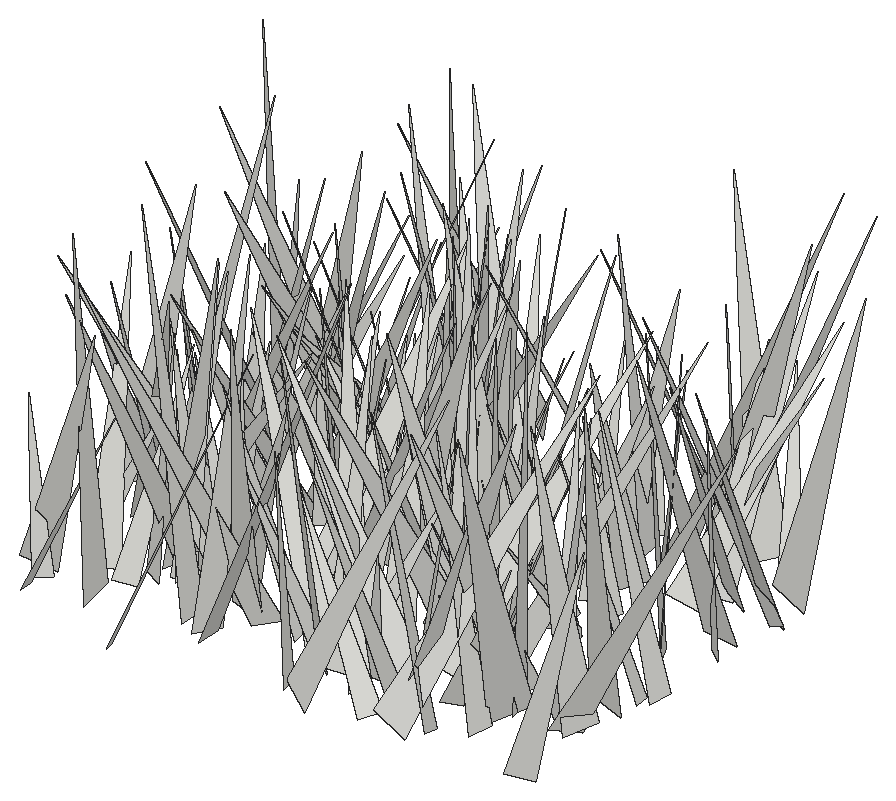
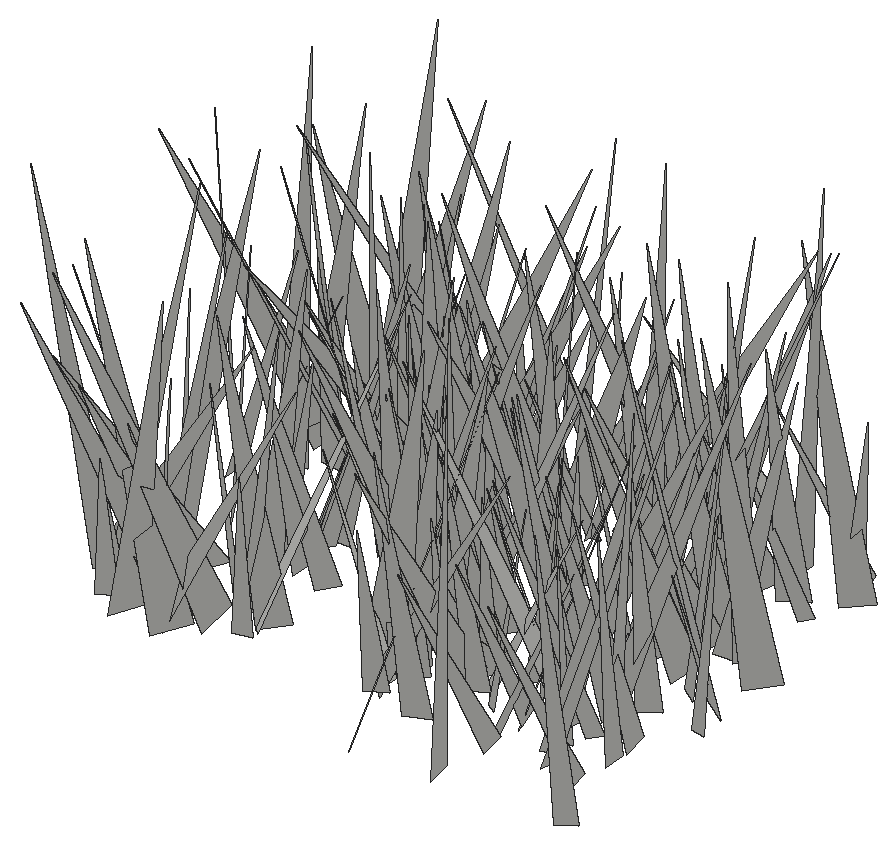
# SketchUp Ruby script. Lengths in inches.
U = 1.inch
M = Sketchup.active_model
def pt(a) = Geom::Point3d.new(a.map { |v| v * U })
def face(e, loops, mat)
  f = e.add_face(loops[0].map { |a| pt(a) })
  loops[1..].each { |l| e.add_face(l.map { |a| pt(a) }).erase! }
  f.material = f.back_material = mat if mat
  f
end
# faces: each face lists its corners as indices into pts; further lists are holes
def faces(e, pts, list, mat = nil) = list.each { |f| face(e, (f[0].is_a?(Array) ? f : [f]).map { |l| l.map { |i| pts[i] } }, mat) }
# xy, xz, yz: faces in a plane at the given z, y or x. An outline is a flat list of corners, or four numbers for a rectangle; further outlines are holes
def ring(l) = l.size == 4 ? [[l[0], l[1]], [l[2], l[1]], [l[2], l[3]], [l[0], l[3]]] : l.each_slice(2).to_a
def flat(e, list, mat, &to3) = list.each { |f| face(e, (f[0].is_a?(Array) ? f : [f]).map { |l| ring(l).map { |u, v| to3.(u, v) } }, mat) }
def xy(e, z, list, mat = nil) = flat(e, list, mat) { |x, y| [x, y, z] }
def xz(e, y, list, mat = nil) = flat(e, list, mat) { |x, z| [x, y, z] }
def yz(e, x, list, mat = nil) = flat(e, list, mat) { |y, z| [x, y, z] }
def lines(e, pts, list) = list.each { |a, b| e.add_line(pt(pts[a]), pt(pts[b])) }
# prism: a flat outline (further loops are holes) pulled along v
def prism(e, loops, v, mat = nil)
  f = face(e, loops, mat); d = Geom::Vector3d.new(v.map { |x| x * U })
  f.pushpull(f.normal.samedirection?(d) ? d.length : -d.length)
end
def box(e, o, s, mat = nil) = prism(e, [[o, [o[0] + s[0], o[1], o[2]], [o[0] + s[0], o[1] + s[1], o[2]], [o[0], o[1] + s[1], o[2]]]], [0, 0, s[2]], mat)
def at(x, y, z, deg = 0) = Geom::Transformation.translation(pt([x, y, z])) * Geom::Transformation.rotation(ORIGIN, Z_AXIS, deg.degrees)
def axes(o, x, y, z) = Geom::Transformation.new([*x, 0, *y, 0, *z, 0, *pt(o).to_a, 1])
def part(name) = M.definitions.add(name)
# library, detail: a bought-in or finely detailed component or shape, given as its bounding box
def library(name, o, s) = part(name).tap { |d| box(d.entities, o, s) }
def detail(e, o, s) = box(e.add_group.entities, o, s)
def put(e, d, t, mat = nil) = e.add_instance(d, t).tap { |i| i.material = mat if mat }
def group(e, t, mat = nil) = e.add_group.tap { |g| g.transformation = t; g.material = mat if mat }.entities
root = M.entities
c1 = part("fur_instance\#9")
p = [[0.8125,0,1.79],[0.67,-0.02,1.48],[0,-0.11,0],[0,0.11,0]]
faces(c1.entities,p,[[0,1,2,3]])
put(root,c1,axes([158.65,304.24,-27.1],[3.34726,-4.07819,1.53745],[-4.35777,-3.09938,1.26621],[0.07255,1.99042,5.12177]))
put(root,c1,axes([134.6875,305.8,-27.1],[2.49015,-6.48815,0.76577],[-6.33726,-2.19962,1.97082],[1.58797,1.39602,6.66429]))
put(root,c1,axes([148.375,303.87,-27.1],[4.07945,6.65627,1.20942],[6.56454,-3.55321,-2.58689],[1.63565,-2.3408,7.36585]))
put(root,c1,axes([147.6,304.41,-27.1],[-4.30965,-1.39305,1.63599],[-1.58025,4.5392,-0.29767],[1.45598,0.80324,4.51941]))
put(root,c1,axes([137.82,305.25,-27.1],[-7.27615,-1.41209,3.18772],[-1.2687,7.94356,0.62294],[3.24745,-0.06052,7.38568]))
put(root,c1,axes([155.44,307.74,-27.1],[6.81384,-4.6319,0.82302],[-4.34734,-6.75311,-2.01405],[-1.7979,-1.22528,7.98915]))
put(root,c1,axes([151.45,304.44,-27.1],[-3.62089,2.64212,0.01483],[2.58278,3.53416,0.96476],[-0.55698,-0.78788,4.37731]))
put(root,c1,axes([151.71,305.8,-27.1],[-0.61117,-4.98438,1.28841],[-4.9544,0.21679,-1.51148],[-1.3993,1.40945,4.78884]))
put(root,c1,axes([147.51,306.48,-27.1],[-4.05006,-5.82532,2.03849],[-5.82326,4.4146,1.04584],[2.04438,1.03428,7.01738]))
put(root,c1,axes([135.48,305.02,-27.1],[-2.21806,2.84038,1.31516],[3.07662,2.27502,0.2754],[0.57601,-1.21396,3.59328]))
put(root,c1,axes([135.39,304.13,-27.1],[4.11341,0.99659,0.14821],[0.94897,-4.04143,0.83763],[-0.33855,0.78037,4.1487]))
put(root,c1,axes([152.29,305.66,-27.1],[5.3173,-1.56529,0.48292],[-1.59322,-5.32309,0.28875],[-0.38078,0.41424,5.53538]))
put(root,c1,axes([140.625,302.53,-27.1],[5.39727,3.08007,0.18691],[2.81936,-5.07536,2.22356],[-1.25418,1.84558,5.80286]))
put(root,c1,axes([149.72,306.74,-27.1],[0.99148,-3.49866,0.36174],[-3.47594,-0.91715,0.65665],[0.53788,0.52224,3.57665]))
put(root,c1,axes([143.02,307.71,-27.1],[-0.95701,-7.3765,1.52863],[-7.35851,1.24531,1.40248],[1.61303,1.30453,7.30491]))
put(root,c1,axes([144.125,307.53,-27.1],[-0.88156,-7.55851,1.51866],[-6.98391,0.13553,-3.37952],[-3.26533,1.75074,6.81814]))
put(root,c1,axes([153.91,304.9375,-27.1],[-5.8174,-1.77979,0.63377],[-1.88895,5.44209,-2.05595],[-0.03436,2.15114,5.72563]))
put(root,c1,axes([154.72,309.3,-27.1],[4.80853,-5.64104,1.01196],[-5.19564,-4.8483,-2.3381],[-2.41883,-0.80002,7.03396]))
put(root,c1,axes([139.82,308.68,-27.1],[0.11863,-7.1905,0.64579],[-7.08435,-0.24031,-1.37429],[-1.39009,0.61104,7.05894]))
put(root,c1,axes([155.33,306.08,-27.1],[-5.94659,0.26274,1.16381],[0.1992,6.05181,-0.34844],[1.17635,0.30341,5.94219]))
put(root,c1,axes([149.81,308.49,-27.1],[-5.8383,-2.13052,1.19785],[-1.77007,5.82456,1.73238],[1.68547,-1.263,5.96857]))
put(root,c1,axes([150.07,305.57,-27.1],[-2.40389,3.30252,0.08348],[3.28439,2.37806,0.4999],[-0.35549,-0.36124,4.05406]))
put(root,c1,axes([153.22,307.02,-27.1],[3.00481,-2.76961,0.12717],[-2.71494,-2.90128,0.96303],[0.56213,0.79222,3.97142]))
put(root,c1,axes([147.14,306.98,-27.1],[-0.30638,-3.92044,1.36874],[-3.76361,-0.31774,-1.75256],[-1.75458,1.36615,3.52026]))
put(root,c1,axes([152.52,305.57,-27.1],[3.86177,3.77021,1.4507],[3.73701,-4.09632,0.69796],[-1.5342,-0.48777,5.35169]))
put(root,c1,axes([151.61,306.74,-27.1],[-6.06762,4.08752,0.30456],[4.00596,5.79855,1.98636],[-0.86766,-1.81261,7.04117]))
put(root,c1,axes([145.65,307.72,-27.1],[-5.30182,-0.75056,0.88287],[-0.65483,5.35184,0.61739],[0.95603,-0.49663,5.31898]))
put(root,c1,axes([141.66,306.17,-27.1],[-7.85501,-1.13743,1.66782],[-1.3997,7.89692,-1.20666],[1.45472,1.45652,7.84468]))
put(root,c1,axes([152.41,304.34,-27.1],[1.49345,8.09623,0.02611],[7.76227,-1.42429,-2.34489],[2.30146,-0.44999,7.89182]))
put(root,c1,axes([143.04,305.375,-27.1],[7.43701,2.08557,1.03262],[1.85087,-7.39668,1.60887],[-1.41074,1.29018,7.55449]))
put(root,c1,axes([142.72,305.72,-27.1],[-6.83852,1.49302,2.47832],[0.97247,7.17644,-1.63995],[2.72497,1.18576,6.80477]))
put(root,c1,axes([158.19,308.45,-27.1],[-6.01027,1.97565,2.91231],[2.62602,6.35479,1.10849],[2.3428,-2.05464,6.22879]))
put(root,c1,axes([141.97,308.67,-27.1],[3.60736,-4.41491,0.21347],[-4.38405,-3.53869,0.89879],[0.56311,0.73233,5.62998]))
put(root,c1,axes([151.7,310.16,-27.1],[1.64942,-7.33453,1.1804],[-6.83961,-1.97125,-2.69132],[-2.89974,0.47759,7.01946]))
put(root,c1,axes([148.56,306.9,-27.1],[0.79551,4.29487,0.6755],[4.10301,-0.51451,-1.56067],[1.4379,-0.90797,4.07959]))
put(root,c1,axes([153.92,309.49,-27.1],[-3.41692,-2.65793,0.41527],[-2.50813,3.39027,1.06197],[0.9728,-0.5949,4.19669]))
put(root,c1,axes([135.52,307.8,-27.1],[0.91676,-3.52562,1.5814],[-3.59518,-0.18259,1.67709],[1.41617,1.81877,3.23385]))
put(root,c1,axes([148.35,306.25,-27.1],[-0.0106,6.43156,0.96228],[6.47441,-0.07994,0.60561],[-0.61077,-0.95901,6.403]))
put(root,c1,axes([138.625,307.6,-27.1],[-2.24155,-3.80564,2.54295],[-4.42537,2.52493,-0.12217],[1.16862,2.26183,4.41503]))
put(root,c1,axes([147.14,307.17,-27.1],[-3.95209,5.35159,0.47213],[5.26841,3.74586,1.6413],[-1.05182,-1.34553,6.44707]))
put(root,c1,axes([136.73,307.01,-27.1],[-2.92394,5.35838,1.35906],[5.44647,3.05552,-0.32925],[0.94614,-1.02969,6.09534]))
put(root,c1,axes([139.3,311.85,-27.1],[-7.53778,-2.79862,0.78068],[-2.32716,7.11502,3.03655],[1.73954,-2.60846,7.44512]))
put(root,c1,axes([157.71,310.46,-27.1],[-1.05079,-7.8114,1.55453],[-7.7743,1.34665,1.51176],[1.73053,1.30661,7.73542]))
put(root,c1,axes([138.09,309.65,-27.1],[-2.71876,-5.31687,1.33657],[-5.469,2.73415,-0.24823],[0.3815,1.3048,5.9665]))
put(root,c1,axes([138.12,306.58,-27.1],[-3.50119,3.09472,0.56001],[2.74674,3.41714,-1.71109],[1.53177,0.94611,4.34831]))
put(root,c1,axes([145.49,307.9,-27.1],[0.85166,3.52496,0.51911],[3.494,-0.72175,-0.83136],[0.69768,-0.68839,3.5298]))
put(root,c1,axes([151.67,310.55,-27.1],[3.93699,-6.31061,2.13001],[-6.14082,-4.39732,-1.67764],[-2.57895,0.83692,7.24632]))
put(root,c1,axes([156.63,308.72,-27.1],[-3.30417,-4.76212,3.2823],[-5.25525,4.05058,0.5865],[2.41528,2.29867,5.7664]))
put(root,c1,axes([138.71,309.0625,-27.1],[6.63487,-1.65212,1.91106],[-1.73662,-6.8834,0.0785],[-1.83462,0.54083,6.83702]))
put(root,c1,axes([139.9,308.95,-27.1],[-4.97089,0.8761,1.32855],[0.91857,5.13772,0.0489],[1.29955,-0.28038,5.04727]))
put(root,c1,axes([148,307.72,-27.1],[4.12915,-1.39251,2.24683],[-2.1688,-4.1671,1.40312],[-1.51116,2.17563,4.12556]))
put(root,c1,axes([151.65,309.99,-27.1],[-5.54142,2.04017,2.02802],[2.50487,5.58649,1.22443],[1.41448,-1.90035,5.77671]))
put(root,c1,axes([139.88,308.18,-27.1],[-3.26703,2.9675,0.38966],[2.97957,3.27925,0.00816],[0.28293,-0.26806,4.41355]))
put(root,c1,axes([135.15,311.64,-27.1],[6.92696,-1.79403,0.01467],[-1.72828,-6.68834,-1.86567],[-0.48147,-1.80253,6.90801]))
put(root,c1,axes([155.5,308.21,-27.1],[-6.71268,-1.89599,2.76742],[-2.51748,6.93875,-1.3526],[2.21714,2.13833,6.8429]))
put(root,c1,axes([139.75,308,-27.1],[0.8824,6.11345,1.2337],[6.18895,-1.01221,0.58924],[-0.77016,-1.12963,6.14863]))
put(root,c1,axes([146.11,308.87,-27.1],[7.40622,-0.19557,0.80001],[-0.28757,-7.3972,0.85392],[-0.77173,0.87956,7.35943]))
put(root,c1,axes([157.79,308.07,-27.1],[6.83257,-2.01041,0.78824],[-2.1593,-6.33413,2.56189],[0.022,2.68032,6.64549]))
put(root,c1,axes([135.98,311.89,-27.1],[1.38462,-5.25865,0.1546],[-5.22749,-1.39323,-0.57157],[-0.5921,0.00308,5.40776]))
put(root,c1,axes([149.4,311.26,-27.1],[3.81645,-5.44593,0.15233],[-5.28758,-3.65777,1.70554],[1.31259,1.09964,6.42764]))
put(root,c1,axes([145.42,310.37,-27.1],[-5.46396,-3.21591,2.3792],[-3.43589,5.83542,-0.00311],[2.04873,1.20967,6.3401]))
put(root,c1,axes([149.63,311.65,-27.1],[-1.836,-5.36618,0.72675],[-5.38286,1.72484,-0.86298],[-0.59066,0.96126,5.60554]))
put(root,c1,axes([152.47,310.41,-27.1],[5.88559,1.89129,2.87248],[1.95642,-6.52369,0.2867],[-2.82853,-0.57687,6.17535]))
put(root,c1,axes([140.24,310.24,-27.1],[-3.96056,0.86775,0.15545],[0.85071,3.94968,-0.37345],[0.23119,0.33194,4.03727]))
put(root,c1,axes([141.125,309.73,-27.1],[-3.9297,0.38452,0.60241],[0.18265,3.7953,-1.23109],[0.69093,1.18368,3.75164]))
put(root,c1,axes([137.38,310.42,-27.1],[4.47757,-3.00826,2.16701],[-3.51648,-4.52249,0.98776],[-1.1747,2.07164,5.30307]))
put(root,c1,axes([153.06,309.27,-27.1],[4.06306,2.1594,0.43468],[1.91332,-3.91175,1.54848],[-1.0914,1.18135,4.33286]))
put(root,c1,axes([156.21,309.74,-27.1],[-0.40963,5.6712,0.85204],[5.69515,0.30195,0.72827],[-0.67361,-0.89587,5.63914]))
put(root,c1,axes([153.89,313.8125,-27.1],[-3.33896,-2.6162,0.26799],[-2.1089,2.92233,2.25332],[1.57125,-1.6372,3.59384]))
put(root,c1,axes([136.96,311.57,-27.1],[4.24231,-3.44067,0.07958],[-3.18347,-3.87509,2.16585],[1.3077,1.72835,5.01442]))
put(root,c1,axes([145.77,310.44,-27.1],[-5.07407,3.61415,0.85454],[3.5922,5.14344,-0.42375],[0.94256,-0.14624,6.2152]))
put(root,c1,axes([158.61,311.51,-27.1],[-4.94313,-1.68267,0.02369],[-1.64372,4.81198,-1.18726],[-0.36076,1.13137,5.08492]))
put(root,c1,axes([149.51,312.18,-27.1],[5.6621,3.46946,2.68851],[3.90579,-5.98471,-0.5026],[-2.00251,-1.86297,6.62147]))
put(root,c1,axes([148.21,310.08,-27.1],[-1.0825,6.58238,0.66021],[6.6005,1.02978,0.55528],[-0.44383,-0.73975,6.64764]))
put(root,c1,axes([145.53,313.68,-27.1],[3.43501,-7.39782,1.03394],[-7.28345,-3.06455,2.27067],[1.65774,1.86463,7.83397]))
put(root,c1,axes([148.88,314.99,-27.1],[3.46816,-3.92613,0.03464],[-3.68547,-3.27126,-1.77763],[-1.35388,-1.15247,4.92774]))
put(root,c1,axes([159.02,312.09,-27.1],[-5.68888,-0.08485,0.69236],[-0.12916,5.71868,-0.36046],[0.68548,0.37338,5.67808]))
put(root,c1,axes([152.85,314.04,-27.1],[1.51534,-5.37644,0.92666],[-5.31705,-1.67082,-0.99923],[-1.22223,0.60275,5.49581]))
put(root,c1,axes([150.66,310.375,-27.1],[5.57667,1.59527,0.3002],[1.43066,-5.3377,1.78788],[-0.76695,1.64269,5.51794]))
put(root,c1,axes([140.3,314.79,-27.1],[-0.06223,-5.95217,0.13196],[-5.73579,0.02457,-1.59678],[-1.59576,0.14382,5.73432]))
put(root,c1,axes([158.22,312.98,-27.1],[-5.21121,-4.35385,3.58957],[-4.50193,6.15376,0.92827],[3.40202,1.4741,6.72689]))
put(root,c1,axes([151.75,310.16,-27.1],[4.07971,3.91858,0.07723],[3.79656,-3.97882,1.32677],[-0.97331,0.90496,5.499]))
put(root,c1,axes([150.89,310.65,-27.1],[-0.59735,8.07244,1.41711],[8.08686,0.34954,1.4177],[-1.33238,-1.49761,7.96939]))
put(root,c1,axes([133.57,312.78,-27.1],[4.4224,-5.22883,1.99199],[-5.58659,-4.26873,1.19762],[-0.31423,2.30295,6.7427]))
put(root,c1,axes([151.49,308.81,-27.1],[-3.48939,6.7058,0.49493],[5.71017,3.24965,-3.77124],[3.55058,1.36403,6.55144]))
put(root,c1,axes([146.32,312.83,-27.1],[-3.33469,1.40616,1.82105],[1.56398,3.73727,-0.02186],[1.68745,-0.685,3.61897]))
put(root,c1,axes([138.22,314.82,-27.1],[2.83348,-4.00549,0.52306],[-3.76222,-2.8494,-1.43972],[-1.47079,-0.42795,4.69039]))
put(root,c1,axes([152.75,311.38,-27.1],[4.68977,6.59581,0.10077],[6.41242,-4.52929,-1.96857],[1.54784,-1.22048,7.85006]))
put(root,c1,axes([146.79,314.75,-27.1],[3.04717,-2.22298,0.43436],[-2.028,-3.00193,-1.13631],[-1.00873,-0.67996,3.59662]))
put(root,c1,axes([152.77,314.59,-27.1],[-4.67386,-0.0885,1.27111],[0.2568,4.66814,1.26925],[1.24804,-1.29194,4.49909]))
put(root,c1,axes([143.4375,313.13,-27.1],[4.00682,1.30969,1.18737],[1.29487,-4.17692,0.23764],[-1.20352,-0.13365,4.20874]))
put(root,c1,axes([146.1,314.22,-27.1],[-4.58905,2.11277,0.48874],[2.15665,4.32669,1.54618],[-0.22698,-1.60562,4.80963]))
put(root,c1,axes([138,313.34,-27.1],[3.18405,-1.52738,1.26596],[-1.78098,-3.25535,0.55182],[-0.87386,1.06936,3.48806]))
put(root,c1,axes([143.01,312.99,-27.1],[-1.4542,4.67664,1.33998],[4.76533,1.65076,-0.58976],[0.97884,-1.08869,4.86188]))
put(root,c1,axes([135.36,314.92,-27.1],[-3.25628,-4.53556,1.56998],[-4.60157,3.48952,0.53691],[1.36443,0.94415,5.55755]))
put(root,c1,axes([153.86,313.7,-27.1],[-3.57996,-1.2077,0.30439],[-1.24532,3.48547,-0.8173],[0.0195,0.87192,3.68872]))
put(root,c1,axes([151.1875,312.91,-27.1],[5.81873,5.70667,1.51485],[5.84557,-5.86726,-0.35074],[-0.83073,-1.31442,8.14252]))
put(root,c1,axes([145.125,314.98,-27.1],[-5.01465,-5.39389,0.78065],[-5.43536,4.87162,-1.25473],[-0.40033,1.42249,7.25716]))
put(root,c1,axes([143.71,311.24,-27.1],[-2.62249,6.7547,0.84995],[6.3246,2.75431,-2.37468],[2.5195,0.11678,6.84575]))
put(root,c1,axes([147.95,313.47,-27.1],[-0.46969,3.55211,0.73396],[3.59032,0.35011,0.60316],[-0.51554,-0.79795,3.53189]))
put(root,c1,axes([141.16,314.57,-27.1],[1.90593,-3.10212,1.28599],[-3.27722,-2.04084,-0.06594],[-0.73267,1.05893,3.64024]))
put(root,c1,axes([136.45,313.76,-27.1],[6.61677,-1.08212,0.53072],[-1.15649,-6.53431,1.0953],[-0.3394,1.16883,6.6146]))
put(root,c1,axes([157.9,317.04,-27.1],[-0.40558,-7.48594,0.6627],[-7.51279,0.42075,0.15485],[0.19107,0.65318,7.49532]))
put(root,c1,axes([138.1875,314.54,-27.1],[2.95558,3.83246,1.3061],[4.0436,-2.87668,-0.7093],[-0.20723,-1.47175,4.78749]))
put(root,c1,axes([148.43,313.5,-27.1],[-6.12572,-2.31991,2.2614],[-2.97153,5.95041,-1.94497],[1.2907,2.68904,6.25488]))
put(root,c1,axes([150.92,313.06,-27.1],[-5.40299,1.91129,1.15946],[1.49374,5.34299,-1.84687],[1.66317,1.41036,5.42535]))
put(root,c1,axes([136.88,317.62,-27.1],[-3.06964,-6.81398,0.3454],[-6.81954,3.05272,-0.38339],[-0.20825,0.47214,7.46364]))
put(root,c1,axes([157.07,314.74,-27.1],[-5.34444,-2.84039,2.21318],[-3.30562,5.4408,-0.99979],[1.42788,1.96442,5.96919]))
put(root,c1,axes([144.86,314.24,-27.1],[1.84734,5.85191,0.92453],[5.8229,-1.61485,-1.41361],[1.09242,-1.28828,5.97153]))
put(root,c1,axes([153.78,315.76,-27.1],[-3.82053,1.38738,1.41647],[1.59253,3.97908,0.39802],[1.18113,-0.87734,4.0451]))
put(root,c1,axes([138.84,317.64,-27.1],[3.08843,-3.08617,0.55459],[-2.71507,-3.02147,-1.69397],[-1.56857,-0.84658,4.0241]))
put(root,c1,axes([140.03,315.78,-27.1],[6.60673,-3.01857,0.44503],[-3.04917,-6.49303,1.22551],[0.11127,1.29906,7.15953]))
put(root,c1,axes([133.3,316.98,-27.1],[-1.38247,-3.90181,0.99129],[-3.91317,1.54858,0.63797],[0.94545,0.70412,4.09003]))
put(root,c1,axes([158.51,315.97,-27.1],[-3.07714,-3.38347,1.94932],[-3.73457,3.27489,-0.21099],[1.14047,1.59489,4.5686]))
put(root,c1,axes([134.58,314.68,-27.1],[1.50713,3.43781,0.3216],[3.3001,-1.53741,0.96906],[-1.01552,0.10596,3.62641]))
put(root,c1,axes([133.91,315.25,-27.1],[-3.45696,-5.56122,4.74392],[-6.59951,4.63089,0.61955],[3.14299,3.60698,6.51874]))
put(root,c1,axes([143.54,314.71,-27.1],[-0.09668,3.9627,0.07364],[3.92699,0.08582,0.53775],[-0.5359,-0.08606,3.92724]))
put(root,c1,axes([152.91,318.16,-27.1],[4.44508,-4.04211,0.97735],[-3.87336,-4.54492,-1.18043],[-1.51359,-0.24009,5.89101]))
put(root,c1,axes([145.24,316.48,-27.1],[-2.81459,-5.30869,2.75415],[-5.79641,3.17103,0.18862],[1.47279,2.33491,6.00571]))
put(root,c1,axes([158.375,319.5625,-27.1],[-2.24137,-6.8028,0.2078],[-6.58087,2.22202,1.76064],[1.73594,-0.35988,6.94277]))
put(root,c1,axes([148.67,314.85,-27.1],[3.62249,2.81644,0.55831],[2.6251,-3.61284,1.19278],[-1.16313,0.61769,4.43081]))
put(root,c1,axes([143.51,315.48,-27.1],[-1.89071,3.52857,0.74513],[3.44423,2.01617,-0.80816],[1.06925,-0.25501,3.92077]))
put(root,c1,axes([146.96,317.48,-27.1],[-6.28621,2.90163,2.83322],[3.4688,6.55463,0.9835],[2.10096,-2.14018,6.85337]))
put(root,c1,axes([135.69,316.86,-27.1],[2.1664,-3.98299,1.68795],[-4.30586,-2.16689,0.41322],[-0.41582,1.68731,4.51516]))
put(root,c1,axes([150.79,316.94,-27.1],[1.73127,-4.9492,1.56465],[-4.93445,-1.0575,2.11492],[1.61056,2.08017,4.79781]))
put(root,c1,axes([140.44,317.72,-27.1],[3.55115,-1.15094,1.45453],[-0.93925,-3.82501,-0.73353],[-1.59941,-0.30919,3.66022]))
put(root,c1,axes([156.45,319.66,-27.1],[-1.98153,-6.18192,0.39554],[-6.00617,2.01899,1.46585],[1.5161,-0.08133,6.32408]))
put(root,c1,axes([148.72,315.67,-27.1],[6.05789,3.57549,2.196],[3.19122,-6.43003,1.66595],[-2.72445,0.41853,6.83424]))
put(root,c1,axes([144.8,317.18,-27.1],[5.13574,3.88277,2.0176],[4.11622,-5.34233,-0.19668],[-1.48436,-1.3806,6.4353]))
put(root,c1,axes([147.13,317.22,-27.1],[-4.91979,-5.33902,1.78444],[-5.59743,4.38767,-2.30455],[-0.5985,2.85253,6.88466]))
put(root,c1,axes([136.66,321.49,-27.1],[-6.90134,-2.30385,2.57209],[-0.73953,6.60101,3.92832],[3.37291,-3.26662,6.12409]))
put(root,c1,axes([138.62,320.89,-27.1],[-4.47086,-3.62986,0.22446],[-3.11938,4.01034,2.72058],[1.8697,-1.98902,5.07572]))
put(root,c1,axes([141.96,317.89,-27.1],[5.92157,-1.3609,0.111],[-1.36516,-5.91048,0.36315],[-0.02664,0.3788,6.06507]))
put(root,c1,axes([136.31,318.0625,-27.1],[2.61538,-3.98544,0.72253],[-3.93735,-2.29982,1.56655],[0.95028,1.43982,4.50221]))
put(root,c1,axes([146.74,315.68,-27.1],[4.8815,3.3845,2.02519],[2.72156,-5.22275,2.16824],[-2.85471,0.80828,5.53015]))
put(root,c1,axes([142.375,317.96,-27.1],[-2.65217,1.9255,1.58872],[2.09556,2.97695,-0.10973],[1.35655,-0.83418,3.2756]))
put(root,c1,axes([146,318.48,-27.1],[0.28341,4.29415,2.46111],[4.89058,0.13603,-0.80051],[0.76092,-2.47364,4.22839]))
put(root,c1,axes([151.11,320.84,-27.1],[-5.31992,-4.92486,0.01845],[-4.88394,5.27914,0.91325],[0.63384,-0.65774,7.19179]))
put(root,c1,axes([139.6875,317.375,-27.1],[3.18185,3.17768,0.5905],[3.1987,-3.21478,0.06397],[-0.46337,-0.37158,4.49642]))
put(root,c1,axes([144.24,320.32,-27.1],[2.99312,-6.69994,0.30324],[-6.59145,-2.87731,1.48788],[1.23852,0.87852,7.18569]))
put(root,c1,axes([152.43,316.27,-27.1],[-4.53148,2.02632,0.31118],[1.79338,4.28391,-1.78018],[0.99329,1.50971,4.63371]))
put(root,c1,axes([139.23,318.82,-27.1],[4.09073,2.15745,2.5023],[2.51133,-4.61824,-0.12369],[-2.14694,-1.2913,4.62314]))
put(root,c1,axes([138.99,321.86,-27.1],[-4.31312,-2.31019,0.44376],[-1.59331,3.55068,2.99849],[1.73068,-2.4885,3.8664]))
put(root,c1,axes([143.48,318.01,-27.1],[6.82569,-2.14516,0.01525],[-2.06759,-6.56497,1.95405],[0.57187,1.86856,6.88284]))
put(root,c1,axes([145.48,316.76,-27.1],[0.70112,8.01126,1.73468],[7.49163,-1.33281,3.12731],[-3.32639,-1.31314,7.4089]))
put(root,c1,axes([137.25,319.14,-27.1],[6.44978,-0.00096,0.92482],[0.04605,-6.50733,-0.32793],[-0.92367,-0.33115,6.44144]))
put(root,c1,axes([144.21,319.72,-27.1],[6.7511,0.38921,2.10678],[0.68602,-6.99103,-0.90679],[-2.02963,-1.06837,6.70124]))
put(root,c1,axes([140.45,320.24,-27.1],[-2.2334,-3.12116,0.78897],[-3.02774,2.36275,0.77617],[1.09405,0.16724,3.75863]))
put(root,c1,axes([141.28,319.32,-27.1],[-3.78552,-3.06993,0.30173],[-3.01727,3.58565,-1.37288],[-0.64154,1.25071,4.67652]))
put(root,c1,axes([158.9375,319.07,-27.1],[-3.53185,-5.19128,1.06072],[-4.89285,2.7062,-3.04713],[-2.03336,2.50511,5.48984]))
put(root,c1,axes([153.37,319.15,-27.1],[3.76786,2.01641,1.4087],[2.07515,-3.9894,0.15999],[-1.32064,-0.51569,4.27049]))
put(root,c1,axes([136.06,319.57,-27.1],[1.52671,4.77623,1.67607],[4.63081,-0.61106,-2.47682],[2.04382,-2.18327,4.35989]))
put(root,c1,axes([141.57,319.59,-27.1],[-0.36242,4.3186,2.109],[4.6668,0.82166,-0.88056],[1.14855,-1.97588,4.24338]))
put(root,c1,axes([145.62,318.38,-27.1],[-3.34888,5.66427,0.75226],[5.70524,3.26636,0.80369],[-0.31635,-1.05439,6.53093]))
put(root,c1,axes([136.09,322.24,-27.1],[-7.13222,-2.21187,1.52983],[-1.72076,7.08542,2.22194],[2.06682,-1.73369,7.12909]))
put(root,c1,axes([138.74,318.17,-27.1],[7.17048,3.0592,0.30714],[3.02615,-7.16002,0.66735],[-0.54355,0.49421,7.76718]))
put(root,c1,axes([136.55,320.62,-27.1],[-1.07299,-3.39329,1.1863],[-3.30809,1.41653,1.05972],[1.4065,0.74301,3.39746]))
put(root,c1,axes([136,318.58,-27.1],[-7.59721,-1.99805,2.32928],[-2.54922,7.5713,-1.81993],[1.70857,2.41215,7.64184]))
put(root,c1,axes([134.52,319.14,-27.1],[5.06172,0.87175,1.3003],[0.68802,-5.19178,0.80241],[-1.40619,0.59773,5.07318]))
put(root,c1,axes([150.53,320.46,-27.1],[-2.5167,4.57974,3.46384],[4.9953,3.61127,-1.14527],[2.83182,-2.30014,5.09864]))
put(root,c1,axes([158,320.93,-27.1],[2.12208,6.92928,3.4126],[7.54208,-1.09525,-2.46604],[1.66665,-3.86645,6.81445]))
put(root,c1,axes([144.57,320.86,-27.1],[4.26627,1.55205,0.05399],[1.49304,-4.05567,-1.39111],[0.42732,-1.32496,4.32143]))
put(root,c1,axes([143.57,318.94,-27.1],[-0.37252,4.33667,0.3989],[4.3129,0.31185,0.63743],[-0.60398,-0.44793,4.30572]))
put(root,c1,axes([153.48,321.51,-27.1],[5.8756,3.65861,0.2575],[3.32747,-5.11292,-3.2803],[1.54262,-2.90637,6.0949]))
put(root,c1,axes([151.75,320.58,-27.1],[-6.14594,-1.15799,1.95321],[-1.28361,6.42082,-0.2323],[1.87305,0.60056,6.24977]))
put(root,c1,axes([134.39,320.57,-27.1],[4.53301,0.32886,1.81446],[0.26511,-4.88148,0.22244],[-1.82486,0.10775,4.53948]))
put(root,c1,axes([145.89,319.67,-27.1],[-3.99948,7.12267,1.32626],[7.23474,3.8453,1.16596],[-0.38726,-1.72292,8.0851]))
put(root,c1,axes([144.88,321.5,-27.1],[-3.87014,-4.65436,0.40491],[-4.4497,3.51193,-2.16136],[-1.42379,1.67578,5.65416]))
put(root,c1,axes([155.11,318.29,-27.1],[-2.23637,5.81255,0.47787],[5.16217,2.21098,-2.73477],[2.71405,0.58421,5.59536]))
put(root,c1,axes([138.96,319.96,-27.1],[3.99187,0.97882,1.10255],[0.50795,-3.90054,1.62373],[-1.38409,1.39155,3.77579]))
put(root,c1,axes([155.06,320.2,-27.1],[0.14678,4.73777,0.12743],[4.7339,-0.15274,0.22615],[-0.23006,-0.12022,4.73465]))
put(root,c1,axes([142.11,319.1,-27.1],[6.07778,0.82962,2.17123],[-0.33597,-5.70106,3.1188],[-2.29992,3.02515,5.28212]))
put(root,c1,axes([151.05,321.71,-27.1],[-1.02276,3.4571,1.0392],[3.60758,1.01767,0.16502],[0.12981,-1.04418,3.60144]))
put(root,c1,axes([154.23,322.66,-27.1],[-4.22462,-4.77942,0.40733],[-4.62488,3.91455,-2.0354],[-1.27248,1.63999,6.04544]))
put(root,c1,axes([154.84,321.88,-27.1],[-3.59286,-3.26733,2.03566],[-3.70516,3.69058,-0.61592],[1.04455,1.85261,4.81713]))
put(root,c1,axes([153.35,323,-27.1],[6.11915,-4.70581,1.11272],[-4.83462,-5.98952,1.25659],[-0.09634,1.67568,7.61641]))
put(root,c1,axes([155.83,319.38,-27.1],[-4.8564,4.18897,0.42907],[3.70643,4.56321,-2.59917],[1.99849,1.71635,5.86314]))
put(root,c1,axes([142.74,325.67,-27.1],[-6.5639,-4.29471,0.69968],[-4.06333,6.50273,1.7952],[1.55674,-1.13527,7.63588]))
put(root,c1,axes([142.13,322.51,-27.1],[-1.06035,5.5551,1.84187],[5.77115,1.30347,-0.60889],[0.97234,-1.67863,5.62252]))
put(root,c1,axes([144.53,321.93,-27.1],[-2.34195,3.99616,0.3444],[3.99913,2.35703,-0.15486],[0.30802,-0.21845,4.62925]))
put(root,c1,axes([152.52,321.37,-27.1],[8.0865,0.10169,1.15451],[-0.2162,-7.86244,2.20681],[-1.13864,2.21504,7.78021]))
put(root,c1,axes([134.52,322.54,-27.1],[4.0884,0.15219,0.34801],[0.0557,-3.96154,1.07814],[-0.37573,1.0688,3.94662]))
put(root,c1,axes([155.5625,322.85,-27.1],[-6.9298,2.98954,1.57704],[3.02348,7.09089,-0.15622],[1.51094,-0.47802,7.54553]))
put(root,c1,axes([156.87,322.47,-27.1],[-2.11834,3.44874,0.2067],[3.45458,2.11778,0.0692],[0.04913,-0.21236,4.04678]))
put(root,c1,axes([138.67,322.4,-27.1],[4.2696,-0.12633,0.87704],[-0.45536,-4.01534,1.6384],[-0.76014,1.6958,3.94476]))
put(root,c1,axes([154.38,321.52,-27.1],[7.47336,0.82298,1.26079],[0.38429,-7.21504,2.43175],[-1.45575,2.3203,7.11442]))
put(root,c1,axes([132.79,325.4,-27.1],[0.54307,-5.39112,1.14857],[-5.29865,-0.1925,1.60174],[1.51911,1.25582,5.17624]))
put(root,c1,axes([138.88,325.3,-27.1],[6.72646,1.81373,2.96578],[2.30607,-7.16166,-0.85049],[-2.60144,-1.65881,6.91459]))
